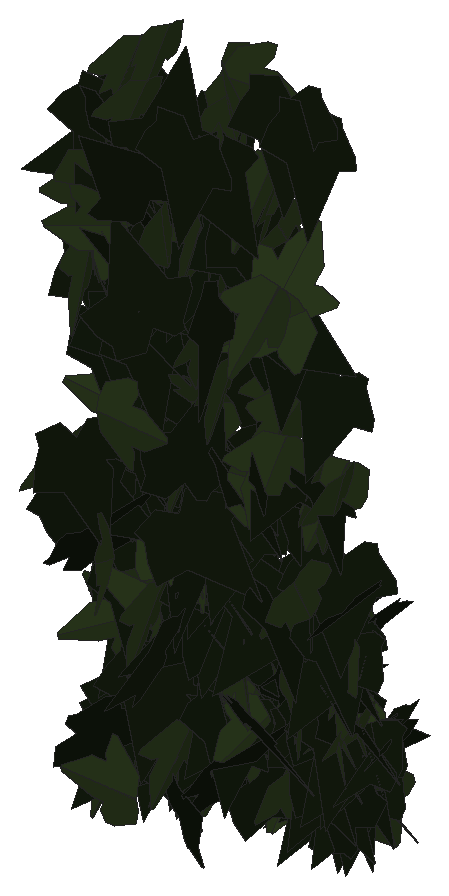
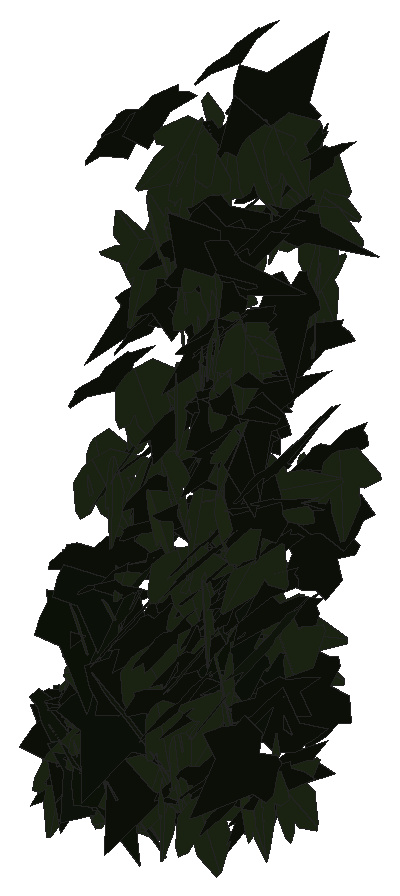
# SketchUp Ruby script. Lengths in inches.
U = 1.inch
M = Sketchup.active_model
def pt(a) = Geom::Point3d.new(a.map { |v| v * U })
def face(e, loops, mat)
  f = e.add_face(loops[0].map { |a| pt(a) })
  loops[1..].each { |l| e.add_face(l.map { |a| pt(a) }).erase! }
  f.material = f.back_material = mat if mat
  f
end
# faces: each face lists its corners as indices into pts; further lists are holes
def faces(e, pts, list, mat = nil) = list.each { |f| face(e, (f[0].is_a?(Array) ? f : [f]).map { |l| l.map { |i| pts[i] } }, mat) }
# xy, xz, yz: faces in a plane at the given z, y or x. An outline is a flat list of corners, or four numbers for a rectangle; further outlines are holes
def ring(l) = l.size == 4 ? [[l[0], l[1]], [l[2], l[1]], [l[2], l[3]], [l[0], l[3]]] : l.each_slice(2).to_a
def flat(e, list, mat, &to3) = list.each { |f| face(e, (f[0].is_a?(Array) ? f : [f]).map { |l| ring(l).map { |u, v| to3.(u, v) } }, mat) }
def xy(e, z, list, mat = nil) = flat(e, list, mat) { |x, y| [x, y, z] }
def xz(e, y, list, mat = nil) = flat(e, list, mat) { |x, z| [x, y, z] }
def yz(e, x, list, mat = nil) = flat(e, list, mat) { |y, z| [x, y, z] }
def lines(e, pts, list) = list.each { |a, b| e.add_line(pt(pts[a]), pt(pts[b])) }
# prism: a flat outline (further loops are holes) pulled along v
def prism(e, loops, v, mat = nil)
  f = face(e, loops, mat); d = Geom::Vector3d.new(v.map { |x| x * U })
  f.pushpull(f.normal.samedirection?(d) ? d.length : -d.length)
end
def box(e, o, s, mat = nil) = prism(e, [[o, [o[0] + s[0], o[1], o[2]], [o[0] + s[0], o[1] + s[1], o[2]], [o[0], o[1] + s[1], o[2]]]], [0, 0, s[2]], mat)
def at(x, y, z, deg = 0) = Geom::Transformation.translation(pt([x, y, z])) * Geom::Transformation.rotation(ORIGIN, Z_AXIS, deg.degrees)
def axes(o, x, y, z) = Geom::Transformation.new([*x, 0, *y, 0, *z, 0, *pt(o).to_a, 1])
def part(name) = M.definitions.add(name)
# library, detail: a bought-in or finely detailed component or shape, given as its bounding box
def library(name, o, s) = part(name).tap { |d| box(d.entities, o, s) }
def detail(e, o, s) = box(e.add_group.entities, o, s)
def put(e, d, t, mat = nil) = e.add_instance(d, t).tap { |i| i.material = mat if mat }
def group(e, t, mat = nil) = e.add_group.tap { |g| g.transformation = t; g.material = mat if mat }.entities
root = M.entities
M.materials.add("efeu1").color = [18, 25, 13]
M.materials.add("efeu2").color = [43, 57, 29]
c1 = part("ivyleaf_9")
p = [[1.54,2.16,1.25],[1.36,2.04,1.19],[-0.21,0.99,0.68],[-0.71,1.11,0.82],[-0.85,0.86,0.67],[-0.8,0.17,0.21],
  [-0.9,-0.01,0.1],[-0.67,-0.16,-0.02],[-0.08,-0.08,-0.05],[-0.03,-0.6,-0.4],[0.65,-0.88,-0.66],[0.83,-0.6,-0.49],
  [1.29,-0.42,-0.43],[1.8125,-0.07,-0.26],[1.21,0.44,0.15]]
faces(c1.entities,p,[[0,1,2,3,4,5,6,7,8,9,10,11,12,13,14]],"efeu1")
c2 = part("ivyleaf_10")
p = [[0,0.5,-0.03],[-0.0625,2.02,-0.43],[-0.19,2.01,-0.46],[-0.54,1.05,-0.29],[-0.52,0.625,-0.18],[-0.83,0.76,-0.28],
  [-1.16,0.64,-0.33],[-1.15,0.33,-0.24],[-0.77,-0.39,0.02],[-0.3,-0.51,0.16],[0.04,-0.48,0.23],[-0.02,2.01,-0.4375],
  [-0.06,2.01,-0.43],[0.04,-0.49,0.23],[0.67,-0.49,0.14],[1.38,0.36,-0.2],[1.375,0.51,-0.24],[0.81,0.65,-0.19],
  [0.62,0.59,-0.15],[0.6,1.09,-0.28],[0.5,1.23,-0.31]]
faces(c2.entities,p,[[0,1,2,3,4,5,6,7,8,9,10],[11,12,0,13,14,15,16,17,18,19,20]],"efeu2")
put(root,c1,axes([9.46,224.35,226.27],[0.2749,-0.41463,-0.05013],[0.01761,0.07147,-0.49455],[0.41728,0.27014,0.05389]))
put(root,c2,axes([10.06,223.54,228.08],[0.14194,0.15824,0.45256],[-0.36519,-0.27011,0.20899],[0.31062,-0.38987,0.0389]))
put(root,c2,axes([9.84,222.3125,228],[-0.06004,-0.49023,-0.07792],[0.009,0.0774,-0.49389],[0.4963,-0.06071,-0.00047]))
put(root,c1,axes([9.97,223.33,231.3],[0.25933,0.14381,-0.40258],[-0.41236,-0.04002,-0.27992],[-0.11274,0.4772,0.09784]))
put(root,c1,axes([9.625,224.54,224.43],[0.44543,0.1332,0.03862],[0.03913,0.00863,-0.45074],[-0.14413,0.41401,-0.00303]))
put(root,c2,axes([9.77,223.57,223.3125],[0.06668,-0.37677,0.32186],[0.11971,-0.3029,-0.37937],[0.48086,0.12766,0.04981]))
put(root,c2,axes([9.8,224.21,227.53],[-0.15262,-0.33669,-0.33667],[0.13993,0.30622,-0.36966],[0.45511,-0.20705,0.00076]))
put(root,c1,axes([9.64,223.48,229.09],[0.0907,-0.48872,0.05409],[0.01102,-0.05297,-0.49706],[0.49158,0.09136,0.00117]))
put(root,c1,axes([10.01,224.11,228.41],[-0.03996,-0.49839,-0.00327],[-0.00499,-0.00288,0.49997],[-0.49838,0.03999,-0.00475]))
put(root,c1,axes([9.9,224.13,225.08],[-0.26591,-0.40496,0.12368],[-0.04722,-0.11678,-0.48387],[0.42078,-0.26902,0.02386]))
put(root,c1,axes([9.95,224.125,228.16],[-0.37783,-0.30014,0.13101],[0.00741,-0.20781,-0.45471],[0.3274,-0.34166,0.16148]))
put(root,c2,axes([10,223.89,223.55],[0.38174,-0.11801,-0.30057],[-0.16042,0.3346,-0.33512],[0.28024,0.3523,0.2176]))
put(root,c1,axes([10.27,223.16,232.22],[-0.43145,-0.0117,0.25242],[-0.24926,-0.06231,-0.42894],[0.04149,-0.49596,0.04793]))
put(root,c2,axes([10.17,222.51,230.97],[-0.29016,0.26632,0.30803],[-0.25874,0.17147,-0.39198],[-0.31442,-0.38688,0.03831]))
put(root,c1,axes([10.04,223.62,223.54],[-0.21327,-0.37981,0.24548],[-0.11457,-0.21717,-0.43556],[0.43748,-0.24203,0.0056]))
put(root,c1,axes([9.85,224.21,227.39],[0.01715,-0.49926,-0.02116],[-0.00077,0.02115,-0.49955],[0.49971,0.01716,-0.00004]))
put(root,c1,axes([9.82,223.78,232.68],[0.10251,-0.48208,-0.08423],[0.0309,0.09226,-0.49044],[0.4884,0.09534,0.0487]))
put(root,c1,axes([10.01,224.09,223.66],[-0.20793,-0.44694,-0.08373],[0.02662,0.07995,-0.49285],[0.45393,-0.20942,-0.00945]))
put(root,c1,axes([9.9375,223.1,230.48],[-0.10726,-0.45007,-0.18955],[0.06748,0.17855,-0.46213],[0.48367,-0.12472,0.02244]))
put(root,c2,axes([10.24,222.44,231.25],[-0.26102,0.32918,0.27113],[-0.21772,0.17047,-0.41658],[-0.36669,-0.33553,0.05434]))
put(root,c1,axes([10.27,223.52,224],[-0.43637,-0.19612,0.14533],[0.12998,0.0653,0.47837],[-0.20662,0.45527,-0.006]))
put(root,c1,axes([9.91,224.15,226.89],[0.03394,-0.45726,-0.19939],[0.06827,0.20223,-0.45215],[0.49415,0.00347,0.07616]))
put(root,c2,axes([10.125,224.01,223.3125],[0.15993,-0.46863,0.06934],[0.03043,-0.06288,-0.4951],[0.47276,0.16258,0.00841]))
put(root,c1,axes([10.39,223.99,229.46],[-0.15758,0.00064,0.47452],[-0.416,-0.24072,-0.13783],[0.22828,-0.43824,0.0764]))
put(root,c2,axes([10.38,223.12,225.52],[-0.06112,-0.05506,0.49319],[-0.23998,-0.43166,-0.07793],[0.43436,-0.24624,0.02634]))
put(root,c2,axes([10.02,223.32,225.35],[-0.42079,-0.14025,0.23078],[0.21949,0.07132,0.44355],[-0.15733,0.4746,0.00155]))
put(root,c2,axes([10.26,222.38,231.86],[-0.44999,-0.21303,0.04608],[-0.03526,-0.03316,-0.49765],[0.21509,-0.45113,0.01481]))
put(root,c1,axes([9.99,223.85,223.4],[0.2056,-0.3836,-0.24613],[-0.09151,0.22977,-0.43455],[0.44649,0.22373,0.02427]))
put(root,c1,axes([9.84,224.17,227.77],[0.0329,-0.11393,0.48573],[0.33799,-0.35298,-0.10569],[0.36699,0.3353,0.05379]))
put(root,c1,axes([10.27,223.41,225.12],[0.32712,0.02137,-0.37754],[-0.37691,0.05871,-0.32325],[0.03051,0.49608,0.05452]))
put(root,c1,axes([9.97,222.35,226.5625],[0.19174,0.46054,-0.03381],[0.00849,0.03308,0.49883],[0.4617,-0.19186,0.00486]))
put(root,c1,axes([10.34,224,229.47],[0.16474,0.3969,-0.2556],[-0.09749,-0.23628,-0.42973],[-0.4619,0.19143,-0.00046]))
put(root,c2,axes([10.11,222.41,230.875],[0.11539,-0.39178,0.28843],[0.20099,-0.23156,-0.39495],[0.44305,0.20709,0.10405]))
put(root,c1,axes([9.97,222.3,227.54],[0.02368,-0.04643,-0.49728],[0.16973,0.46895,-0.0357],[0.46971,-0.16711,0.03797]))
put(root,c2,axes([10.28,223.11,233.51],[0.00004,-0.46731,0.17782],[0.01933,-0.17769,-0.46696],[0.49963,0.00692,0.01805]))
put(root,c2,axes([10.29,223.91,230.61],[-0.14528,-0.46695,-0.10415],[0.0252,0.10123,-0.489],[0.47776,-0.14733,-0.00588]))
put(root,c1,axes([10.1,222.26,228.24],[0.06508,-0.45194,-0.20375],[-0.03871,0.20024,-0.45652],[0.49423,0.07519,-0.00892]))
put(root,c1,axes([10.39,223.99,229.59],[0.23931,0.27184,-0.34472],[-0.21889,-0.26645,-0.36207],[-0.38055,0.3242,-0.00852]))
put(root,c1,axes([10.08,223.43,225.84],[0.03578,-0.48607,0.11161],[0.01574,-0.11074,-0.48733],[0.49847,0.03838,0.00738]))
put(root,c1,axes([10.16,224.49,223.47],[-0.02313,-0.46595,0.17989],[-0.02184,-0.17896,-0.46636],[0.49899,-0.02943,-0.01207]))
put(root,c1,axes([10.07,223.46,226.21],[0.00968,-0.38062,-0.32409],[0.11352,0.31736,-0.36932],[0.48685,-0.06643,0.09257]))
put(root,c2,axes([10.65,223.9,230.35],[0.03888,0.03318,0.49738],[-0.4528,-0.20629,0.04915],[0.20847,-0.45425,0.01401]))
put(root,c2,axes([10.36,223.22,224.04],[0.26877,-0.36634,-0.20871],[-0.0635,0.20951,-0.44953],[0.41681,0.26814,0.0661]))
put(root,c2,axes([10.375,223.58,233.51],[-0.00984,-0.48491,0.12151],[-0.00138,-0.12151,-0.48501],[0.4999,-0.00988,0.00105]))
put(root,c1,axes([10.2,224.03,226.52],[-0.04338,-0.4978,0.01768],[0.00042,-0.01778,-0.49968],[0.49811,-0.04334,0.00197]))
put(root,c2,axes([10.3125,224.06,229.17],[-0.13039,0.47123,0.1046],[-0.01596,0.10408,-0.48879],[-0.48244,-0.1308,-0.0121]))
put(root,c2,axes([10.48,223.95,229.8],[-0.14744,-0.45851,0.13428],[-0.00766,-0.13824,-0.48045],[0.47771,-0.14373,0.03374]))
put(root,c1,axes([10.35,222.67,232.875],[-0.17141,-0.4553,0.11541],[0.00417,-0.12432,-0.48428],[0.46968,-0.16505,0.04641]))
put(root,c2,axes([10.43,222.84,232.52],[0.09858,-0.43178,-0.23205],[0.06241,0.24582,-0.4309],[0.4862,0.05599,0.10236]))
put(root,c1,axes([10.32,223.83,230.35],[-0.03922,-0.42596,0.25888],[0.06014,-0.26183,-0.4217],[0.49482,-0.00194,0.07177]))
put(root,c1,axes([10.3,222.1,224.23],[0.05558,0.27081,-0.41662],[0.04888,0.41421,0.27576],[0.49449,-0.07138,0.01956]))
put(root,c1,axes([10.27,224.39,225.1],[0.24515,-0.43359,-0.04361],[-0.01057,0.0441,-0.49794],[0.43565,0.24506,0.01246]))
put(root,c1,axes([10.29,224.0625,229.11],[0.14125,-0.3605,-0.31637],[0.02248,0.33441,-0.37103],[0.47911,0.09059,0.11068]))
put(root,c1,axes([10.35,224.06,229.5],[-0.18648,-0.25656,-0.38653],[0.24482,0.29944,-0.31686],[0.39407,-0.30744,0.01395]))
put(root,c1,axes([10.6,223.89,229.61],[-0.29837,-0.37269,0.1486],[-0.06415,-0.13849,-0.47614],[0.39606,-0.30319,0.03482]))
put(root,c2,axes([10.6,224.53,223.12],[-0.15077,-0.45723,0.13492],[0.01976,-0.14738,-0.47738],[0.47632,-0.13862,0.06251]))
put(root,c1,axes([10.47,223.55,224.86],[-0.34493,-0.08293,-0.35234],[0.34178,0.08566,-0.35475],[0.1192,-0.48558,-0.00241]))
put(root,c1,axes([10.99,223.79,231.49],[-0.28866,0.07585,0.40115],[-0.39028,0.09292,-0.2984],[-0.11982,-0.4854,0.00556]))
put(root,c1,axes([10.36,223.72,226.79],[0.45577,-0.19877,-0.05253],[-0.04839,0.02045,-0.49723],[0.19982,0.45834,-0.0006]))
put(root,c2,axes([10.66,222.77,233.18],[-0.01889,-0.47699,0.14874],[-0.01438,-0.14827,-0.47729],[0.49944,-0.02231,-0.00812]))
put(root,c1,axes([10.49,222.83,229.93],[-0.08128,-0.48391,-0.09605],[0.01321,0.09517,-0.49068],[0.49317,-0.0823,-0.00269]))
put(root,c1,axes([10.51,223.91,230.83],[-0.14138,-0.44313,-0.18343],[0.03722,0.18052,-0.46479],[0.47815,-0.14508,-0.01805]))
put(root,c2,axes([10.93,223.66,224.68],[-0.01131,0.09649,0.49047],[-0.42458,0.25707,-0.06037],[-0.26382,-0.41786,0.07612]))
put(root,c1,axes([11,223.8,231.72],[-0.01933,0.01637,0.49936],[-0.46278,0.18778,-0.02407],[-0.18832,-0.46311,0.0079]))
put(root,c2,axes([10.64,224.38,226.5625],[0.31281,-0.37862,-0.09381],[0.02059,0.1361,-0.48068],[0.38952,0.29686,0.10074]))
put(root,c1,axes([10.36,222.61,232.86],[0.23886,-0.41401,0.14679],[0.10521,-0.1083,-0.47666],[0.42647,0.25859,0.03537]))
put(root,c2,axes([10.37,224.21,224.83],[0.04188,-0.09028,0.49],[0.45696,-0.18901,-0.07388],[0.19857,0.45401,0.06667]))
put(root,c2,axes([10.6875,221.98,232.56],[-0.45077,-0.18289,-0.11556],[0.10845,0.04006,-0.48645],[0.18719,-0.46362,0.00355]))
put(root,c1,axes([10.61,224.44,223.64],[-0.14975,-0.41675,0.23214],[0.02153,-0.24897,-0.43307],[0.47656,-0.11971,0.09251]))
put(root,c2,axes([10.6,223.92,224.53],[0.20865,0.37218,0.26066],[0.07787,0.2533,-0.424],[-0.44766,0.21753,0.04774]))
put(root,c2,axes([10.72,223.82,227.83],[0.11615,-0.43541,0.21663],[0.07574,-0.20381,-0.45025],[0.48039,0.13741,0.01862]))
put(root,c2,axes([11.08,221.63,231.96],[0.1724,-0.01883,-0.46896],[-0.46084,0.08784,-0.17294],[0.0889,0.49186,0.01293]))
put(root,c1,axes([10.47,223.6,225.43],[0.49015,-0.05469,0.08224],[0.08249,-0.00231,-0.49314],[0.05432,0.49699,0.00676]))
put(root,c2,axes([10.88,223.54,228.49],[0.02454,0.03782,-0.49796],[-0.07931,0.49253,0.0335],[0.49306,0.07734,0.03017]))
put(root,c2,axes([10.77,223.44,226.02],[-0.46164,-0.16327,-0.10112],[0.09194,0.04325,-0.48957],[0.16862,-0.47061,-0.00991]))
put(root,c1,axes([10.59,222.86,230.44],[0.20234,-0.40855,-0.20529],[-0.04609,0.20513,-0.45365],[0.4549,0.20251,0.04536]))
put(root,c1,axes([11.15,223.7,232.125],[-0.2717,-0.23934,-0.34481],[-0.21893,-0.26964,0.35967],[-0.35812,0.34643,0.04172]))
put(root,c2,axes([10.79,223.81,230.39],[0.14106,-0.44262,-0.18491],[0.04398,0.20386,-0.45443],[0.47767,0.11194,0.09645]))
put(root,c2,axes([10.49,223.69,223.11],[0.08876,-0.18521,0.45587],[0.42581,-0.20323,-0.16548],[0.24659,0.4176,0.12165]))
put(root,c2,axes([10.79,222.9,225.96],[0.10138,-0.44337,0.20771],[0.07537,-0.19546,-0.454],[0.48378,0.12337,0.0272]))
put(root,c1,axes([10.64,222.94,229.8],[0.07908,-0.49345,-0.01575],[-0.0017,0.01568,-0.49975],[0.4937,0.0791,0.0008]))
put(root,c1,axes([10.59,224.27,227.3],[0.25231,-0.38843,-0.18832],[-0.00237,0.21688,-0.45051],[0.43166,0.22823,0.1076]))
put(root,c2,axes([11.03,221.67,227.18],[0.15391,-0.24517,-0.40768],[-0.21924,0.34371,-0.28947],[0.42219,0.26787,-0.0017]))
put(root,c1,axes([10.76,223.91,230.53],[-0.12673,-0.44819,0.18184],[0.01289,-0.19104,-0.46188],[0.4835,-0.11238,0.05998]))
put(root,c1,axes([10.8,223.05,224.91],[-0.15429,-0.4746,-0.03082],[0.00529,0.03069,-0.49903],[0.47557,-0.15432,-0.00445]))
put(root,c2,axes([10.93,223.9,230.9375],[0.29053,-0.35642,-0.19635],[-0.00995,0.23497,-0.44124],[0.40681,0.26029,0.12944]))
put(root,c1,axes([10.78,224.05,226.11],[-0.00685,-0.49132,0.09252],[-0.01701,-0.09225,-0.49112],[0.49966,-0.00987,-0.01545]))
put(root,c1,axes([10.7,223.92,230.58],[0.15498,-0.35377,-0.31753],[0.01916,0.33836,-0.36762],[0.47499,0.10178,0.11844]))
put(root,c2,axes([11,223.78,231.6875],[-0.19672,-0.45961,0.00758],[-0.00206,-0.00737,-0.49994],[0.45967,-0.19673,0.001]))
put(root,c1,axes([10.72,224.4,225.67],[0.30045,-0.3736,-0.14196],[-0.04708,0.14329,-0.47671],[0.39688,0.29982,0.05093]))
put(root,c1,axes([10.83,222.89,229.43],[0.01915,-0.29529,-0.40303],[-0.01066,0.403,-0.29577],[0.49952,0.01992,0.00914]))
put(root,c1,axes([10.82,224.3125,223.68],[0.03998,-0.46685,-0.1745],[-0.00683,0.17453,-0.4685],[0.49835,0.03984,0.00758]))
put(root,c1,axes([10.99,223.68,226.07],[0.23056,-0.03816,-0.44203],[-0.31486,0.33689,-0.19331],[0.31258,0.36749,0.13131]))
put(root,c2,axes([11.05,223.85,231.07],[-0.2631,-0.42363,0.03622],[0.01256,-0.05033,-0.4973],[0.42499,-0.26077,0.03713]))
put(root,c2,axes([11.06,224.48,223.9],[0.14211,-0.46758,-0.10569],[-0.01573,0.10563,-0.48846],[0.47912,0.14215,0.01531]))
put(root,c1,axes([10.95,223.82,231.56],[-0.20039,-0.12365,0.44108],[0.37354,0.23458,0.23546],[-0.26517,0.42389,-0.00164]))
put(root,c2,axes([10.8,223.21,226.71],[0.40168,0.1281,0.26878],[0.2501,0.09976,-0.4213],[-0.16157,0.4729,0.01606]))
put(root,c1,axes([11.35,223.52,225.9],[-0.06305,0.29901,0.39575],[-0.21991,0.34073,-0.29247],[-0.4446,-0.21094,0.08854]))
put(root,c2,axes([11.17,224.28,226.82],[-0.33727,-0.33915,0.14569],[-0.0474,-0.15592,-0.4727],[0.36606,-0.33266,0.07302]))
put(root,c1,axes([10.98,224,226.43],[-0.08948,-0.46537,0.15946],[-0.02059,-0.1584,-0.4738],[0.4915,-0.09136,0.00918]))
put(root,c2,axes([11.45,221.49,224.07],[0.00565,0.02496,0.49934],[-0.49357,-0.07936,0.00955],[0.07974,-0.49303,0.02374]))
put(root,c2,axes([11.14,222.6,231.65],[0.04787,-0.45772,-0.19544],[0.01425,0.19753,-0.45911],[0.4975,0.03838,0.03196]))
put(root,c1,axes([10.93,224.3,225.48],[0.10688,-0.45151,-0.18633],[-0.02092,0.18633,-0.46351],[0.488,0.10687,0.02094]))
put(root,c2,axes([11.13,223.86,227.61],[0.04968,-0.43934,-0.23347],[0.04021,0.23741,-0.4382],[0.4959,0.02476,0.05893]))
put(root,c1,axes([11.07,223.32,226.78],[-0.38574,-0.06389,-0.31164],[0.30378,0.07146,-0.39066],[0.09445,-0.49073,-0.01631]))
put(root,c2,axes([11.14,223.91,230.58],[0.26444,-0.41222,-0.10071],[0.01084,0.12519,-0.48395],[0.42421,0.25377,0.07515]))
put(root,c1,axes([11.25,223.59,225.58],[-0.10239,-0.07618,-0.48344],[0.10531,-0.48577,0.05424],[-0.47794,-0.09071,0.11552]))
put(root,c2,axes([11.13,223.63,226.52],[-0.07591,0.47126,0.14882],[-0.05673,0.14127,-0.47626],[-0.49094,-0.08919,0.03202]))
put(root,c1,axes([10.96,223.97,227.19],[0.15351,-0.47366,-0.04555],[0.00818,0.05049,-0.49738],[0.47578,0.15196,0.02325]))
put(root,c1,axes([10.77,223.9,230.71],[0.18582,-0.10335,0.45254],[0.38299,-0.24129,-0.21237],[0.26228,0.42556,-0.01051]))
put(root,c2,axes([11.54,223.16,228.9],[0.11457,0.18019,-0.45211],[-0.48624,0.06243,-0.09834],[0.02101,0.46221,0.18954]))
put(root,c1,axes([11,224.56,224.79],[0.12304,-0.4833,-0.03575],[0.00353,0.03778,-0.49856],[0.48461,0.12244,0.01271]))
put(root,c1,axes([11,224.11,224.5],[0.13772,-0.45951,-0.14102],[0.00235,0.14734,-0.47779],[0.48065,0.13094,0.04275]))
put(root,c2,axes([11.26,224.6,224.42],[0.02348,-0.49936,-0.00939],[0.0004,0.00942,-0.49991],[0.49945,0.02346,0.00084]))
put(root,c2,axes([11.06,223.5625,224.14],[-0.29047,-0.22054,-0.34204],[0.29668,0.1729,-0.36344],[0.27858,-0.41408,0.03042]))
put(root,c2,axes([11.27,224.45,223.27],[0.12072,-0.42198,-0.23951],[-0.01662,0.24307,-0.43663],[0.48492,0.11338,0.04465]))
put(root,c1,axes([10.86,223.63,225.44],[0.24298,-0.29184,0.32525],[0.23812,-0.22362,-0.37854],[0.36641,0.33886,0.03032]))
put(root,c1,axes([11,223.23,232.08],[0.33812,-0.28831,-0.22923],[-0.05118,0.27138,-0.41682],[0.36476,0.30534,0.154]))
put(root,c2,axes([11.33,222.83,224.23],[-0.00124,-0.45942,0.19732],[0.00656,-0.19732,-0.45937],[0.49996,0.00145,0.00652]))
put(root,c2,axes([11.42,223.05,232.62],[-0.45035,0.16672,0.13926],[-0.12887,0.053,-0.48019],[-0.17488,-0.4684,-0.00476]))
put(root,c1,axes([11.3125,222.49,232.58],[-0.30955,-0.1955,0.34053],[0.30638,0.15094,0.36517],[-0.24558,0.43474,0.02634]))
put(root,c1,axes([11.27,224.55,224.89],[-0.22947,-0.44182,-0.04624],[0.01767,0.04293,-0.49784],[0.44388,-0.23011,-0.00408]))
put(root,c2,axes([11.35,223.73,225.9],[-0.10127,-0.45139,-0.1897],[0.04144,0.18512,-0.46262],[0.48788,-0.10942,-0.00008]))
put(root,c2,axes([11.37,223.66,232.86],[-0.09963,-0.46573,-0.15222],[0.06066,0.14242,-0.47543],[0.4862,-0.1132,0.02812]))
put(root,c2,axes([11.4,224.03,229.63],[0.18033,-0.43214,-0.17531],[-0.00172,0.18735,-0.46357],[0.46635,0.1678,0.06608]))
put(root,c1,axes([11.37,221.73,231.31],[0.30741,-0.39427,0.00695],[-0.00265,0.00674,0.49995],[-0.39432,-0.30742,0.00205]))
put(root,c1,axes([11.21,224.45,225.82],[0.12093,-0.47164,-0.11371],[-0.02546,0.11086,-0.48689],[0.48449,0.12355,0.0028]))
put(root,c2,axes([11.61,223.97,228.04],[0.24302,-0.18753,-0.39468],[-0.26326,0.29762,-0.30351],[0.34876,0.35533,0.04592]))
put(root,c1,axes([11.37,223.67,226.07],[-0.28605,-0.39438,-0.11243],[0.06599,0.09102,-0.4872],[0.40474,-0.29357,-0.00002]))
put(root,c1,axes([11.07,223.72,226.24],[0.17544,-0.34479,0.31677],[0.20128,-0.24988,-0.38347],[0.42274,0.26207,0.05112]))
put(root,c2,axes([11.26,224.71,223.55],[0.45478,0.11715,0.1716],[0.15338,0.08927,-0.46744],[-0.14016,0.47781,0.04526]))
put(root,c2,axes([11.5,223.59,233.38],[-0.22919,0.40197,0.18944],[-0.09516,0.16382,-0.46272],[-0.43407,-0.24816,0.00141]))
put(root,c2,axes([11.29,223.05,231.17],[0.08698,-0.14188,0.47149],[0.30207,-0.36272,-0.16488],[0.38883,0.31353,0.02261]))
put(root,c1,axes([11.25,222.88,223.03],[-0.01796,-0.05304,0.49685],[0.20583,-0.45382,-0.041],[0.45532,0.20306,0.03813]))
put(root,c2,axes([11.54,223.86,231.19],[0.29828,-0.38694,-0.10633],[0.00162,0.13365,-0.4818],[0.40128,0.28708,0.08098]))
put(root,c1,axes([11.41,223.42,225.78],[0.06438,-0.29072,-0.40166],[-0.07332,0.395,-0.29765],[0.49039,0.09723,0.00823]))
put(root,c1,axes([11.52,223.79,224.39],[-0.26747,-0.37472,0.19506],[0.02448,-0.24423,-0.43561],[0.42174,-0.22347,0.14899]))
put(root,c2,axes([11.66,224.4,225.09],[-0.23704,-0.37413,0.23204],[-0.05207,-0.23786,-0.4367],[0.43715,-0.2312,0.0738]))
put(root,c1,axes([11.53,224.62,223.71],[0.32517,0.37905,-0.02416],[-0.01074,-0.02261,-0.49937],[-0.37967,0.32528,-0.00656]))
put(root,c2,axes([11.2,221.62,229.3],[0.01327,-0.00456,-0.4998],[0.45524,-0.20631,0.01397],[-0.20635,-0.45543,-0.00133]))
put(root,c1,axes([11.54,222.62,228.09],[-0.22656,-0.18696,0.40462],[0.3387,0.22284,0.29262],[-0.28975,0.40668,0.02567]))
put(root,c2,axes([11.64,222.93,230.16],[0.09399,-0.48981,-0.03533],[-0.0046,0.03509,-0.49875],[0.49106,0.09408,0.00209]))
put(root,c2,axes([11.48,223.65,233.33],[-0.17283,-0.22775,-0.4102],[0.25355,0.32248,-0.28587],[0.39477,-0.30682,0.00402]))
put(root,c1,axes([11.45,223.92,229.08],[0.08819,-0.46339,-0.16582],[-0.01334,0.16615,-0.4714],[0.49198,0.08757,0.01694]))
put(root,c1,axes([11.39,222.75,227.41],[0.07927,-0.28377,-0.40397],[0.09472,0.41028,-0.26962],[0.4845,-0.03378,0.11881]))
put(root,c1,axes([11.5,223.87,231.04],[-0.06182,-0.47292,-0.1501],[0.02256,0.14842,-0.47693],[0.49565,-0.06574,0.00299]))
put(root,c2,axes([11.66,224.79,223.19],[0.29952,0.3463,-0.2009],[-0.12846,-0.15451,-0.45785],[-0.37919,0.32589,-0.00359]))
put(root,c1,axes([11.83,221.49,232.69],[0.18486,0.06394,0.46015],[-0.42411,-0.17892,0.19524],[0.18963,-0.46249,-0.01192]))
put(root,c2,axes([11.73,224.16,227.61],[0.19258,-0.45937,0.04344],[0.00733,-0.04402,-0.498],[0.46137,0.19245,-0.01022]))
put(root,c1,axes([11.7,223.5625,227.28],[-0.32149,-0.36814,-0.10542],[0.06744,0.08107,-0.48875],[0.37695,-0.32848,-0.00247]))
put(root,c1,axes([12.07,224.65,224.51],[-0.31298,0.32756,0.21154],[-0.15747,0.14197,-0.45282],[-0.35672,-0.35007,0.01429]))
put(root,c1,axes([11.72,224.26,227.37],[-0.24089,-0.42202,0.11777],[0.02567,-0.14776,-0.47698],[0.43739,-0.22376,0.09285]))
put(root,c1,axes([11.57,223.46,224.24],[0.00191,-0.46131,0.19285],[0.0739,-0.19047,-0.45635],[0.4945,0.03025,0.06746]))
put(root,c2,axes([11.8,223.11,229.48],[0.12657,-0.47646,0.08343],[0.03252,-0.07767,-0.49286],[0.48262,0.13019,0.01133]))
put(root,c1,axes([11.61,224.38,225.83],[0.14036,-0.40239,-0.2615],[-0.04947,0.25887,-0.4249],[0.47734,0.14516,0.03286]))
put(root,c1,axes([11.625,223.4,228.07],[0.33916,-0.33853,-0.14273],[-0.10843,0.09336,-0.47909],[0.35102,0.35592,-0.01008]))
put(root,c1,axes([11.67,222.8125,223.58],[0.06369,0.47442,-0.14447],[-0.00631,0.14642,0.47804],[0.49589,-0.05907,0.02464]))
put(root,c2,axes([11.81,223.65,224.16],[-0.16317,-0.07282,0.46698],[0.15047,-0.47633,-0.0217],[0.44804,0.13345,0.17735]))
put(root,c1,axes([11.74,223.94,227.9],[0.09401,-0.44067,-0.21672],[-0.04778,0.2114,-0.45058],[0.48875,0.10543,-0.00237]))
put(root,c1,axes([11.78,223.8,223.44],[0.04167,-0.0951,-0.4891],[-0.01725,0.49024,-0.09679],[0.49796,0.02494,0.03757]))
put(root,c1,axes([12,224.6875,224.37],[0.21356,0.44603,0.07382],[-0.00846,0.08557,-0.49255],[-0.45202,0.20912,0.0441]))
put(root,c1,axes([12.17,221.13,231.16],[-0.36118,-0.3184,0.1348],[0.1028,0.08724,0.48148],[-0.33012,0.37552,0.00245]))
put(root,c1,axes([12.24,224.52,223.28],[-0.3855,0.31812,-0.01375],[0.011,-0.00826,-0.49981],[-0.31823,-0.38566,-0.00063]))
put(root,c1,axes([11.82,223.5,231.51],[0.08526,-0.45151,-0.19716],[-0.00883,0.19866,-0.45876],[0.4926,0.0817,0.0259]))
put(root,c1,axes([11.96,224.46,224.5625],[0.22891,0.27658,0.348],[-0.24517,-0.24796,0.35834],[0.3708,-0.33469,0.0221]))
put(root,c1,axes([12.27,224.7,223.33],[-0.1794,0.46139,-0.07024],[-0.03262,-0.08746,-0.49121],[-0.46556,-0.17167,0.06148]))
put(root,c2,axes([12.0625,223.77,231.96],[0.24516,-0.43523,0.02166],[0.01429,-0.01681,-0.49951],[0.43553,0.24554,0.0042]))
put(root,c2,axes([12.11,222.47,232.98],[0.25681,-0.42345,-0.06883],[-0.0349,0.05933,-0.49524],[0.42759,0.25917,0.00092]))
put(root,c2,axes([11.99,223.27,227.95],[0.04739,0.22702,0.44296],[0.04062,0.44172,-0.23073],[-0.49609,0.05786,0.02342]))
put(root,c2,axes([12.11,223.8,231.29],[-0.04507,-0.41198,-0.27972],[0.05142,0.27552,-0.41406],[0.4953,-0.06609,0.01754]))
put(root,c2,axes([12.11,224.58,223.49],[0.07804,-0.46123,0.17656],[0.02982,-0.17403,-0.46779],[0.49297,0.08354,0.00034]))
put(root,c1,axes([11.96,222.48,232.81],[0.07623,-0.35781,-0.34082],[-0.05727,0.33613,-0.3657],[0.49082,0.09479,0.01027]))
put(root,c2,axes([11.82,223.25,225.38],[0.22252,-0.13339,0.42742],[0.38987,-0.17701,-0.25821],[0.2202,0.44819,0.02523]))
put(root,c2,axes([12.22,223.89,229.22],[-0.13855,-0.45826,0.14422],[-0.00898,-0.1476,-0.47763],[0.48034,-0.13494,0.03267]))
put(root,c2,axes([12.18,224.6,223.53],[0.16063,-0.47349,-0.00164],[0.00975,0.00504,-0.49988],[0.4734,0.16056,0.01085]))
put(root,c1,axes([12.2,223.3125,228.38],[0.23732,-0.13496,-0.41888],[-0.33439,0.2541,-0.27132],[0.28611,0.40892,0.03034]))
put(root,c1,axes([12.14,224.3125,223.36],[0.25554,0.33292,0.27177],[0.0983,0.26252,-0.41403],[-0.41837,0.26503,0.06872]))
put(root,c1,axes([12,224.48,225.66],[0.17637,-0.46782,-0.00585],[0.005,0.00814,-0.49991],[0.46783,0.17628,0.00755]))
put(root,c1,axes([12.35,224.62,223.35],[-0.48106,-0.08301,-0.10813],[0.10427,0.03145,-0.488],[0.08782,-0.49206,-0.01295]))
put(root,c2,axes([12.21,223.34,232.31],[-0.05304,-0.37812,0.32282],[0.11009,-0.32553,-0.3632],[0.48484,0.03255,0.11778]))
put(root,c2,axes([12.32,224.54,224.08],[-0.11174,-0.4649,0.14623],[0.00021,-0.15007,-0.47695],[0.48735,-0.10653,0.03373]))
put(root,c1,axes([12.33,223.54,226.16],[-0.32482,-0.36268,0.11381],[-0.04263,-0.114,-0.48496],[0.37772,-0.32476,0.04313]))
put(root,c2,axes([12.33,223.72,228.86],[-0.0507,-0.37224,0.32995],[0.01224,-0.33249,-0.37323],[0.49727,-0.02977,0.04283]))
put(root,c1,axes([12.53,220.91,226.6875],[-0.35772,0.34535,-0.05263],[0.0338,-0.04077,-0.49719],[-0.3477,-0.35926,0.00582]))
put(root,c1,axes([12.43,224.75,223.18],[0.12038,0.31811,0.36649],[-0.05436,0.38406,-0.31551],[-0.48224,0.03612,0.12705]))
put(root,c1,axes([12.21,223.8,228.11],[-0.12843,-0.42267,0.23421],[0.02862,-0.24857,-0.43289],[0.48238,-0.09778,0.08804]))
put(root,c2,axes([12.42,223.69,224.74],[0.34211,-0.28097,-0.2324],[-0.10162,0.23259,-0.43079],[0.35019,0.34199,0.10204]))
put(root,c2,axes([12.39,223.68,223.63],[-0.12373,-0.41476,-0.25034],[0.07052,0.2402,-0.43282],[0.47929,-0.14241,-0.00095]))
put(root,c1,axes([12.11,224.67,223.73],[0.25759,-0.4241,0.06155],[0.03645,-0.04987,-0.49617],[0.42699,0.2601,0.00522]))
put(root,c1,axes([12.29,222.32,230.9375],[-0.31548,0.00088,-0.38791],[0.38534,-0.05672,-0.31352],[-0.04456,-0.49677,0.03511]))
put(root,c2,axes([12.44,223.33,228.44],[-0.20266,-0.40327,0.21517],[0.03366,-0.2479,-0.43291],[0.45584,-0.16098,0.12763]))
put(root,c2,axes([12.48,224.63,223.66],[-0.13436,-0.48161,0.00112],[0.00022,-0.00123,-0.5],[0.48161,-0.13436,0.00054]))
put(root,c1,axes([12.41,224.62,223.59],[-0.21111,-0.43324,0.13318],[-0.05499,-0.12135,-0.48192],[0.4499,-0.21813,0.00359]))
put(root,c1,axes([12.21,224.32,224.32],[0.22857,-0.37953,-0.23177],[-0.05854,0.23264,-0.43869],[0.44083,0.22768,0.06191]))
put(root,c2,axes([12.55,224.11,224.1],[-0.47388,0.14481,0.06683],[-0.07559,-0.01945,-0.49387],[-0.14044,-0.47817,0.04032]))
put(root,c2,axes([12.47,224.16,227.79],[0.13952,-0.45498,-0.1534],[0.0237,0.16607,-0.47102],[0.47956,0.12416,0.0679]))
put(root,c1,axes([12.25,224.33,224.09],[0.03151,-0.47289,-0.15933],[0.06095,0.1621,-0.46905],[0.49527,0.01014,0.06786]))
put(root,c2,axes([12.54,224.47,223.32],[-0.26706,-0.42271,-0.00005],[0.00572,-0.00355,-0.49995],[0.42267,-0.26703,0.00673]))
put(root,c1,axes([12.35,223.58,230.14],[0.03746,-0.48664,0.10855],[0.00454,-0.10851,-0.48806],[0.49857,0.03755,-0.00371]))
put(root,c1,axes([12.39,221.67,233.57],[-0.03815,-0.48493,0.11568],[0.02928,-0.118,-0.48499],[0.49768,-0.03023,0.0374]))
put(root,c1,axes([12.47,224.78,223.49],[-0.15708,-0.46898,-0.0734],[0.00814,0.07464,-0.49433],[0.47462,-0.15649,-0.01581]))
put(root,c2,axes([12.59,224.56,223.95],[-0.28121,0.39565,0.11991],[-0.07485,0.0939,-0.48537],[-0.40659,-0.29093,0.00642]))
put(root,c1,axes([12.43,223.25,230.39],[0.15683,-0.17102,-0.4429],[-0.10132,0.44363,-0.20718],[0.46383,0.15473,0.10449]))
put(root,c2,axes([12.54,224.55,223.78],[0.3915,0.30841,0.04012],[-0.05445,0.13146,-0.47933],[-0.30621,0.37094,0.13652]))
put(root,c1,axes([12.88,224.73,223.6],[-0.39215,0.30731,0.04218],[-0.03713,0.02101,-0.49818],[-0.30797,-0.39385,0.00634]))
put(root,c2,axes([12.67,224.25,227.77],[-0.19048,-0.40264,0.22716],[-0.00554,-0.24368,-0.43657],[0.46226,-0.16883,0.08837]))
put(root,c1,axes([12.31,224.34,225.48],[0.32636,-0.37568,0.04846],[0.06715,-0.00556,-0.49544],[0.3728,0.32989,0.04683]))
put(root,c1,axes([12.68,224.67,223.79],[0.19612,0.45672,-0.0543],[-0.01562,-0.05238,-0.497],[-0.45967,0.19664,-0.00628]))
put(root,c2,axes([12.9,222.91,230.7],[0.24562,0.09978,-0.42393],[-0.41088,-0.10828,-0.26354],[-0.1444,0.47783,0.0288]))
put(root,c1,axes([12.37,223.43,226.1],[0.11245,-0.42538,0.23751],[0.11322,-0.21426,-0.43735],[0.47385,0.15215,0.04814]))
put(root,c1,axes([12.52,223.47,233.41],[-0.09005,-0.48901,-0.05251],[0.01506,0.05062,-0.4972],[0.49159,-0.09113,0.00561]))
put(root,c2,axes([12.66,223.43,226.51],[-0.09416,-0.42838,-0.24005],[0.07013,0.23019,-0.43829],[0.48602,-0.11621,0.01673]))
put(root,c1,axes([12.43,224.77,223.4375],[0.15801,-0.47284,0.03816],[0.00631,-0.03813,-0.4985],[0.47433,0.15802,-0.00609]))
put(root,c1,axes([13.05,224.04,223.07],[-0.11056,0.07348,0.48205],[-0.4117,0.25081,-0.13266],[-0.2613,-0.42626,0.00504]))
put(root,c2,axes([12.66,224.4375,224.33],[-0.3643,0.34214,-0.01494],[0.01043,-0.01072,-0.49978],[-0.34231,-0.36445,0.00067]))
put(root,c2,axes([12.53,224.14,224.42],[-0.33139,0.24122,-0.28635],[0.18848,-0.22293,-0.40593],[-0.32351,-0.37698,0.05682]))
put(root,c1,axes([12.85,224.48,225.55],[-0.02599,0.4993,0.00469],[-0.02635,0.00332,-0.49929],[-0.49863,-0.0262,0.02614]))
put(root,c2,axes([12.75,224.44,223.93],[0.37117,-0.30069,-0.1477],[-0.09254,0.11984,-0.47652],[0.32198,0.38108,0.03331]))
put(root,c1,axes([12.59,224.74,223.47],[-0.08605,-0.49254,0.00155],[0.00578,-0.00259,-0.49996],[0.49251,-0.08602,0.00613]))
put(root,c2,axes([12.76,224.24,224.52],[0.15125,-0.21634,0.42464],[-0.16825,0.39259,0.25994],[-0.44588,-0.22153,0.04596]))
put(root,c1,axes([12.61,224.6,223.76],[0.39372,0.17729,0.25209],[-0.22659,-0.11069,0.43175],[0.2089,-0.45422,-0.00681]))
put(root,c2,axes([12.67,224.6875,223.67],[-0.03733,0.46994,0.16661],[-0.0177,0.16573,-0.4714],[-0.49829,-0.04109,0.00426]))
put(root,c2,axes([12.65,224.14,224.63],[0.24793,0.43115,-0.05139],[-0.02412,-0.04541,-0.49735],[-0.43353,0.24909,-0.00171]))
put(root,c1,axes([12.47,224.56,223.59],[0.482,-0.13202,-0.01557],[-0.01411,0.0074,-0.49975],[0.13219,0.4822,0.00341]))
put(root,c1,axes([12.48,224.14,227.82],[0.1642,-0.44191,0.1666],[0.05465,-0.15742,-0.47142],[0.4691,0.17302,-0.0034]))
put(root,c1,axes([12.53,224.04,223.77],[0.2101,-0.40227,-0.20984],[-0.04091,0.21351,-0.45027],[0.45187,0.20637,0.0568]))
put(root,c2,axes([12.68,224.65,223.75],[0.18968,-0.37818,0.26646],[0.11825,-0.23879,-0.42308],[0.44726,0.22352,-0.00115]))
put(root,c1,axes([12.8,224.69,223.5],[-0.338,-0.36761,0.02484],[-0.00808,-0.02631,-0.49924],[0.36836,-0.33789,0.01184]))
put(root,c1,axes([12.92,224.02,226.02],[-0.04214,0.49692,-0.03593],[-0.00225,-0.03625,-0.49868],[-0.49822,-0.04186,0.00529]))
put(root,c2,axes([12.61,223.2,230.85],[0.46699,0.06741,-0.16545],[0.14505,0.12724,0.46127],[0.10429,-0.47882,0.09928]))
put(root,c1,axes([12.53,222.45,225.1875],[0.48712,-0.10676,-0.03632],[-0.0353,0.00856,-0.49868],[0.1071,0.48839,0.0008]))
put(root,c1,axes([12.71,224.3125,226.58],[-0.2036,-0.42293,-0.17226],[0.07547,0.15485,-0.46939],[0.45039,-0.21714,0.00078]))
put(root,c1,axes([12.86,224.1875,224.37],[-0.12737,-0.2145,0.43332],[0.22452,0.37062,0.24945],[-0.42821,0.25813,0.00191]))
put(root,c2,axes([12.85,222.6,231.03],[-0.13114,-0.32641,0.35533],[0.08903,-0.37827,-0.31462],[0.47421,-0.01925,0.15734]))
put(root,c1,axes([12.59,224.54,223.85],[0.23086,-0.44305,-0.02016],[0.03308,0.03986,-0.49731],[0.44228,0.22829,0.04772]))
put(root,c1,axes([12.77,224.1,229.26],[-0.10868,-0.4698,0.1322],[-0.01192,-0.13284,-0.48188],[0.4879,-0.1079,0.01768]))
put(root,c1,axes([12.85,224.62,224.13],[-0.26666,-0.41894,0.05815],[0.017,-0.0793,-0.49338],[0.42261,-0.26116,0.05654]))
put(root,c1,axes([13.15,224.63,224.06],[-0.32897,0.37236,-0.05595],[-0.03189,-0.10158,-0.48853],[-0.37518,-0.31786,0.09058]))
put(root,c1,axes([12.98,224.49,224.25],[-0.38271,-0.31959,0.03728],[-0.0368,-0.01408,-0.49845],[0.31965,-0.38427,-0.01274]))
put(root,c2,axes([12.9,224.51,225.5],[0.31925,-0.38314,-0.03592],[-0.02044,0.02972,-0.4987],[0.38427,0.31988,0.00331]))
put(root,c2,axes([12.92,223.92,227.86],[0.07107,-0.49492,0.00199],[-0.00148,-0.00222,-0.49999],[0.49492,0.07106,-0.00178]))
put(root,c2,axes([12.93,224.28,224.25],[-0.03797,-0.48035,-0.13351],[0.00004,0.13389,-0.48174],[0.49856,-0.03659,-0.01013]))
put(root,c1,axes([12.94,224.1,225.64],[-0.35681,-0.34939,0.02474],[-0.00455,-0.03069,-0.49904],[0.35023,-0.35635,0.01873]))
put(root,c1,axes([12.82,224.3,224.37],[-0.14721,-0.47754,0.01703],[-0.0035,-0.01675,-0.49971],[0.47783,-0.14724,0.00159]))
put(root,c1,axes([12.79,223.62,233.06],[-0.01394,-0.4988,0.0317],[-0.01517,-0.03128,-0.49879],[0.49958,-0.01487,-0.01426]))
put(root,c1,axes([12.97,224.37,224.14],[-0.30071,-0.3795,0.12474],[-0.01313,-0.14666,-0.47783],[0.39925,-0.29065,0.07824]))
put(root,c1,axes([12.72,224.1,224.8125],[0.42657,-0.2419,-0.09756],[-0.07699,0.06192,-0.49014],[0.24922,0.43318,0.01558]))
put(root,c2,axes([12.93,224,225.48],[0.44183,-0.23375,-0.01199],[-0.01059,0.00562,-0.49986],[0.23382,0.44196,0.00002]))
put(root,c2,axes([12.97,224.6875,223.14],[-0.12493,-0.44906,-0.18094],[0.06016,0.17102,-0.46598],[0.48039,-0.13819,0.0113]))
put(root,c2,axes([13.02,224.4,224.12],[-0.30252,0.3724,0.14071],[-0.10163,0.09862,-0.47953],[-0.38491,-0.31873,0.01603]))
put(root,c1,axes([12.8,224.08,225.86],[0.01323,-0.49209,-0.0876],[0.01109,0.08789,-0.49209],[0.4997,0.01108,0.01324]))
